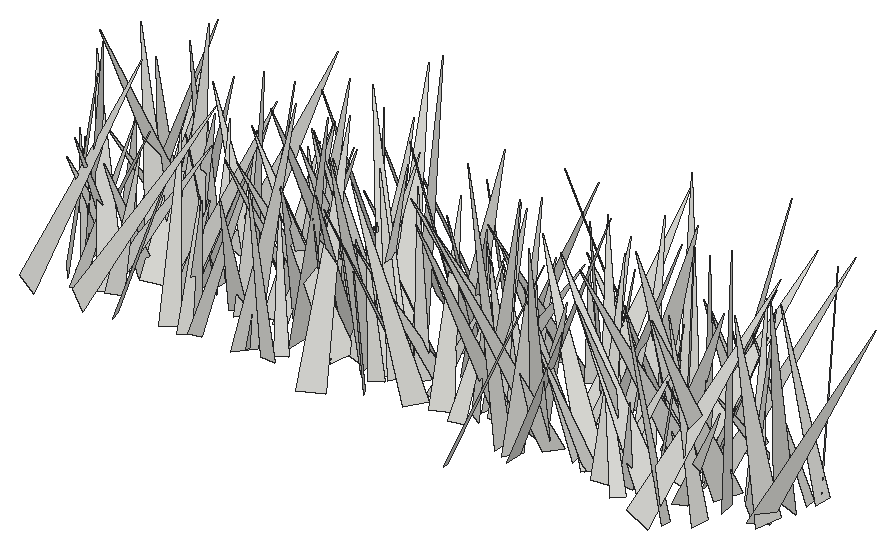
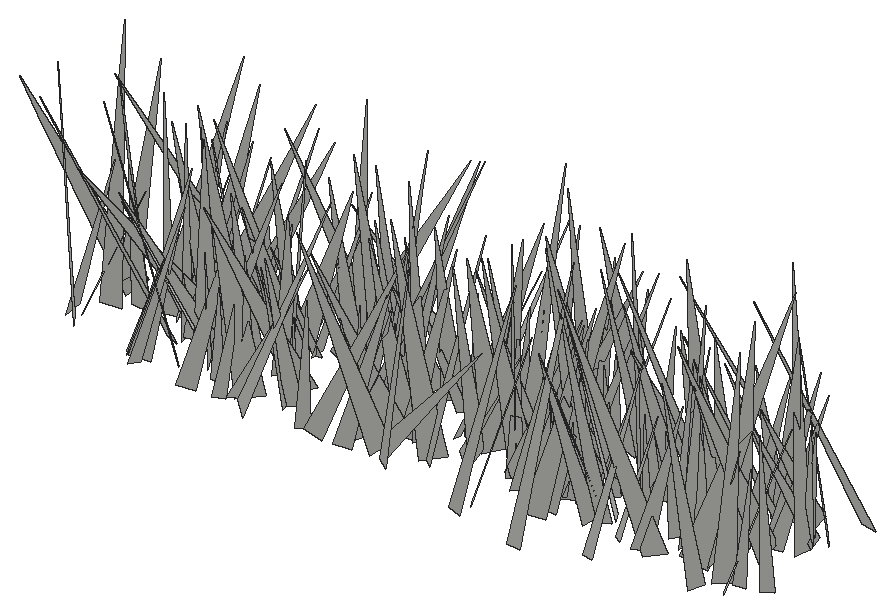
# SketchUp Ruby script. Lengths in inches.
U = 1.inch
M = Sketchup.active_model
def pt(a) = Geom::Point3d.new(a.map { |v| v * U })
def face(e, loops, mat)
  f = e.add_face(loops[0].map { |a| pt(a) })
  loops[1..].each { |l| e.add_face(l.map { |a| pt(a) }).erase! }
  f.material = f.back_material = mat if mat
  f
end
# faces: each face lists its corners as indices into pts; further lists are holes
def faces(e, pts, list, mat = nil) = list.each { |f| face(e, (f[0].is_a?(Array) ? f : [f]).map { |l| l.map { |i| pts[i] } }, mat) }
# xy, xz, yz: faces in a plane at the given z, y or x. An outline is a flat list of corners, or four numbers for a rectangle; further outlines are holes
def ring(l) = l.size == 4 ? [[l[0], l[1]], [l[2], l[1]], [l[2], l[3]], [l[0], l[3]]] : l.each_slice(2).to_a
def flat(e, list, mat, &to3) = list.each { |f| face(e, (f[0].is_a?(Array) ? f : [f]).map { |l| ring(l).map { |u, v| to3.(u, v) } }, mat) }
def xy(e, z, list, mat = nil) = flat(e, list, mat) { |x, y| [x, y, z] }
def xz(e, y, list, mat = nil) = flat(e, list, mat) { |x, z| [x, y, z] }
def yz(e, x, list, mat = nil) = flat(e, list, mat) { |y, z| [x, y, z] }
def lines(e, pts, list) = list.each { |a, b| e.add_line(pt(pts[a]), pt(pts[b])) }
# prism: a flat outline (further loops are holes) pulled along v
def prism(e, loops, v, mat = nil)
  f = face(e, loops, mat); d = Geom::Vector3d.new(v.map { |x| x * U })
  f.pushpull(f.normal.samedirection?(d) ? d.length : -d.length)
end
def box(e, o, s, mat = nil) = prism(e, [[o, [o[0] + s[0], o[1], o[2]], [o[0] + s[0], o[1] + s[1], o[2]], [o[0], o[1] + s[1], o[2]]]], [0, 0, s[2]], mat)
def at(x, y, z, deg = 0) = Geom::Transformation.translation(pt([x, y, z])) * Geom::Transformation.rotation(ORIGIN, Z_AXIS, deg.degrees)
def axes(o, x, y, z) = Geom::Transformation.new([*x, 0, *y, 0, *z, 0, *pt(o).to_a, 1])
def part(name) = M.definitions.add(name)
# library, detail: a bought-in or finely detailed component or shape, given as its bounding box
def library(name, o, s) = part(name).tap { |d| box(d.entities, o, s) }
def detail(e, o, s) = box(e.add_group.entities, o, s)
def put(e, d, t, mat = nil) = e.add_instance(d, t).tap { |i| i.material = mat if mat }
def group(e, t, mat = nil) = e.add_group.tap { |g| g.transformation = t; g.material = mat if mat }.entities
root = M.entities
c1 = part("fur_instance\#9")
p = [[0.8125,0,1.79],[0.67,-0.02,1.48],[0,-0.11,0],[0,0.11,0]]
faces(c1.entities,p,[[0,1,2,3]])
put(root,c1,axes([140.625,446.28,-27.1],[5.39727,3.08007,0.18691],[2.81936,-5.07536,2.22356],[-1.25418,1.84558,5.80286]))
put(root,c1,axes([116.41,447.99,-27.1],[4.19181,1.99584,0.5753],[1.88629,-4.2003,0.82769],[-0.86965,0.50967,4.56832]))
put(root,c1,axes([125.84,449.39,-27.1],[-1.40726,-4.75955,2.034],[-5.17479,1.24906,-0.65748],[-0.10975,2.13481,4.91949]))
put(root,c1,axes([113.78,448.04,-27.1],[4.07618,6.66518,0.05677],[6.29765,-3.82934,-2.59208],[2.18344,-1.39809,7.37028]))
put(root,c1,axes([149.72,450.49,-27.1],[0.99148,-3.49866,0.36174],[-3.47594,-0.91715,0.65665],[0.53788,0.52224,3.57665]))
put(root,c1,axes([143.02,451.46,-27.1],[-0.95701,-7.3765,1.52863],[-7.35851,1.24531,1.40248],[1.61303,1.30453,7.30491]))
put(root,c1,axes([119.95,450.31,-27.1],[3.72524,-2.31212,0.81738],[-2.32656,-3.80205,-0.15146],[-0.77532,0.29988,4.38182]))
put(root,c1,axes([120.54,448.8,-27.1],[-2.95191,2.4359,0.97471],[2.3622,3.10602,-0.60836],[1.1418,-0.12828,3.77853]))
put(root,c1,axes([110.49,447.77,-27.1],[3.27574,7.01328,0.4286],[6.91428,-3.13335,-1.57325],[1.25002,-1.04703,7.57902]))
put(root,c1,axes([144.125,451.28,-27.1],[-0.88156,-7.55851,1.51866],[-6.98391,0.13553,-3.37952],[-3.26533,1.75074,6.81814]))
put(root,c1,axes([133.73,452.16,-27.1],[-4.47092,-4.93614,0.16266],[-4.90041,4.46105,0.68268],[0.61475,-0.33851,6.62484]))
put(root,c1,axes([153.91,448.6875,-27.1],[-5.8174,-1.77979,0.63377],[-1.88895,5.44209,-2.05595],[-0.03436,2.15114,5.72563]))
put(root,c1,axes([114.86,449.83,-27.1],[-2.17172,3.54056,2.13295],[3.72846,2.71807,-0.7156],[1.78427,-1.37037,4.09143]))
put(root,c1,axes([154.72,453.05,-27.1],[4.80853,-5.64104,1.01196],[-5.19564,-4.8483,-2.3381],[-2.41883,-0.80002,7.03396]))
put(root,c1,axes([139.82,452.43,-27.1],[0.11863,-7.1905,0.64579],[-7.08435,-0.24031,-1.37429],[-1.39009,0.61104,7.05894]))
put(root,c1,axes([130.49,452.47,-27.1],[7.53052,-1.13144,2.64431],[-0.30654,-7.68469,-2.41514],[-2.85982,-2.15562,7.22191]))
put(root,c1,axes([119.4,448.99,-27.1],[3.60121,-2.60608,3.3834],[-3.59297,-4.24118,0.55747],[-2.30861,2.53545,4.41017]))
put(root,c1,axes([155.33,449.83,-27.1],[-5.94659,0.26274,1.16381],[0.1992,6.05181,-0.34844],[1.17635,0.30341,5.94219]))
put(root,c1,axes([132.16,449.81,-27.1],[-3.20539,-1.99252,1.2784],[-2.28309,3.17085,-0.78241],[0.62603,1.36182,3.69222]))
put(root,c1,axes([149.81,452.24,-27.1],[-5.8383,-2.13052,1.19785],[-1.77007,5.82456,1.73238],[1.68547,-1.263,5.96857]))
put(root,c1,axes([135.17,450.52,-27.1],[-3.75455,5.21199,1.89568],[5.51913,3.28609,1.89629],[-0.5456,-2.62523,6.13723]))
put(root,c1,axes([150.07,449.32,-27.1],[-2.40389,3.30252,0.08348],[3.28439,2.37806,0.4999],[-0.35549,-0.36124,4.05406]))
put(root,c1,axes([153.22,450.77,-27.1],[3.00481,-2.76961,0.12717],[-2.71494,-2.90128,0.96303],[0.56213,0.79222,3.97142]))
put(root,c1,axes([147.14,450.73,-27.1],[-0.30638,-3.92044,1.36874],[-3.76361,-0.31774,-1.75256],[-1.75458,1.36615,3.52026]))
put(root,c1,axes([152.52,449.32,-27.1],[3.86177,3.77021,1.4507],[3.73701,-4.09632,0.69796],[-1.5342,-0.48777,5.35169]))
put(root,c1,axes([151.61,450.49,-27.1],[-6.06762,4.08752,0.30456],[4.00596,5.79855,1.98636],[-0.86766,-1.81261,7.04117]))
put(root,c1,axes([124.23,449.36,-27.1],[6.87844,-2.02965,2.77665],[-2.6588,-7.07628,1.41394],[-2.18175,2.22463,7.03088]))
put(root,c1,axes([111.28,450.27,-27.1],[4.60486,4.04407,1.88978],[4.30358,-4.74303,-0.33665],[-1.18533,-1.50984,6.1193]))
put(root,c1,axes([113.47,452.25,-27.1],[-0.2394,-4.99537,0.47277],[-5.01072,0.21306,-0.28607],[-0.26442,0.48521,4.99291]))
put(root,c1,axes([129.92,448,-27.1],[-5.97227,4.9002,0.90124],[4.6479,5.98621,-1.7477],[1.79477,0.80344,7.52499]))
put(root,c1,axes([145.65,451.47,-27.1],[-5.30182,-0.75056,0.88287],[-0.65483,5.35184,0.61739],[0.95603,-0.49663,5.31898]))
put(root,c1,axes([111.55,452.125,-27.1],[7.9282,0.66664,2.15118],[1.11346,-8.00329,-1.62351],[-1.9576,-1.85234,7.78877]))
put(root,c1,axes([141.66,449.92,-27.1],[-7.85501,-1.13743,1.66782],[-1.3997,7.89692,-1.20666],[1.45472,1.45652,7.84468]))
put(root,c1,axes([114.93,452.67,-27.1],[3.23703,-3.40023,0.62778],[-3.13183,-3.24768,-1.44163],[-1.46538,-0.57015,4.46784]))
put(root,c1,axes([112.91,452.87,-27.1],[3.29812,-3.00828,0.87507],[-2.53709,-3.30998,-1.81667],[-1.83812,-0.82908,4.07763]))
put(root,c1,axes([121.28,452.55,-27.1],[1.53045,-4.60076,0.23907],[-4.60681,-1.52625,0.11946],[0.03806,0.26453,4.84716]))
put(root,c1,axes([152.41,448.09,-27.1],[1.49345,8.09623,0.02611],[7.76227,-1.42429,-2.34489],[2.30146,-0.44999,7.89182]))
put(root,c1,axes([114.52,449.98,-27.1],[-3.46559,5.8146,1.30946],[5.95968,3.40104,0.67057],[0.08042,-1.46897,6.73574]))
put(root,c1,axes([126.2,450.12,-27.1],[-1.47936,3.73163,0.54523],[3.76451,1.42617,0.45319],[-0.22551,-0.67216,3.98851]))
put(root,c1,axes([143.04,449.125,-27.1],[7.43701,2.08557,1.03262],[1.85087,-7.39668,1.60887],[-1.41074,1.29018,7.55449]))
put(root,c1,axes([142.72,449.47,-27.1],[-6.83852,1.49302,2.47832],[0.97247,7.17644,-1.63995],[2.72497,1.18576,6.80477]))
put(root,c1,axes([158.19,452.2,-27.1],[-6.01027,1.97565,2.91231],[2.62602,6.35479,1.10849],[2.3428,-2.05464,6.22879]))
put(root,c1,axes([128.33,451.64,-27.1],[-3.06281,-3.15709,1.43812],[-3.29391,3.24851,0.11628],[1.08883,0.94666,4.3971]))
put(root,c1,axes([127.84,454.125,-27.1],[-0.91329,-6.82842,0.06821],[-6.63421,0.90353,1.6239],[1.61843,-0.14959,6.69511]))
put(root,c1,axes([112.84,449.09,-27.1],[4.59265,0.40937,1.72839],[-0.43371,-4.3881,2.19176],[-1.72245,2.19644,4.05662]))
put(root,c1,axes([125.98,452.01,-27.1],[7.89082,-0.9052,1.78608],[-0.78265,-8.07818,-0.63641],[-1.84308,-0.44515,7.91703]))
put(root,c1,axes([141.97,452.42,-27.1],[3.60736,-4.41491,0.21347],[-4.38405,-3.53869,0.89879],[0.56311,0.73233,5.62998]))
put(root,c1,axes([151.7,453.91,-27.1],[1.64942,-7.33453,1.1804],[-6.83961,-1.97125,-2.69132],[-2.89974,0.47759,7.01946]))
put(root,c1,axes([113.76,451.03,-27.1],[3.2036,5.15972,0.63397],[4.7617,-2.61371,-2.78969],[2.08586,-1.95793,5.39475]))
put(root,c1,axes([131.92,451.17,-27.1],[-1.38179,3.78074,1.32931],[4.00762,1.30133,0.46468],[-0.00636,-1.40818,3.99842]))
put(root,c1,axes([112.24,450.73,-27.1],[0.5553,3.90242,1.15183],[3.90207,-0.84018,0.96535],[-1.15302,-0.96393,3.8217]))
put(root,c1,axes([117.9,451.76,-27.1],[1.20072,-3.47995,0.99765],[-3.52529,-0.88496,1.15597],[0.82322,1.28603,3.49507]))
put(root,c1,axes([111.97,451.16,-27.1],[0.50374,3.60666,1.32904],[3.78488,-0.69911,0.46265],[-0.67011,-1.23747,3.61216]))
put(root,c1,axes([128.89,452.07,-27.1],[-6.43604,2.78332,0.65453],[2.85741,6.20344,1.71766],[-0.1023,-1.83529,6.79846]))
put(root,c1,axes([148.56,450.65,-27.1],[0.79551,4.29487,0.6755],[4.10301,-0.51451,-1.56067],[1.4379,-0.90797,4.07959]))
put(root,c1,axes([124.49,454.31,-27.1],[6.011,-2.52803,0.45147],[-2.2406,-5.7244,-2.22212],[-1.25478,-1.8887,6.13068]))
put(root,c1,axes([153.92,453.24,-27.1],[-3.41692,-2.65793,0.41527],[-2.50813,3.39027,1.06197],[0.9728,-0.5949,4.19669]))
put(root,c1,axes([134.04,453.875,-27.1],[-4.91943,-1.92287,0.32626],[-1.70701,4.67316,1.80343],[0.9434,-1.57124,4.96446]))
put(root,c1,axes([135.52,451.55,-27.1],[0.91676,-3.52562,1.5814],[-3.59518,-0.18259,1.67709],[1.41617,1.81877,3.23385]))
put(root,c1,axes([148.35,450,-27.1],[-0.0106,6.43156,0.96228],[6.47441,-0.07994,0.60561],[-0.61077,-0.95901,6.403]))
put(root,c1,axes([138.625,451.35,-27.1],[-2.24155,-3.80564,2.54295],[-4.42537,2.52493,-0.12217],[1.16862,2.26183,4.41503]))
put(root,c1,axes([126.09,454.23,-27.1],[4.34994,-4.04005,0.73934],[-3.73736,-4.34022,-1.72779],[-1.70317,-0.79441,5.67968]))
put(root,c1,axes([147.14,450.92,-27.1],[-3.95209,5.35159,0.47213],[5.26841,3.74586,1.6413],[-1.05182,-1.34553,6.44707]))
put(root,c1,axes([121.12,449,-27.1],[5.49101,0.89671,2.25711],[-0.37206,-5.20349,2.97239],[-2.40004,2.85822,4.70322]))
put(root,c1,axes([136.73,450.76,-27.1],[-2.92394,5.35838,1.35906],[5.44647,3.05552,-0.32925],[0.94614,-1.02969,6.09534]))
put(root,c1,axes([139.3,455.6,-27.1],[-7.53778,-2.79862,0.78068],[-2.32716,7.11502,3.03655],[1.73954,-2.60846,7.44512]))
put(root,c1,axes([124.3,449.85,-27.1],[-6.72177,-1.11045,3.37602],[-2.29516,6.87097,-2.30972],[2.71346,3.06096,6.4094]))
put(root,c1,axes([157.71,454.21,-27.1],[-1.05079,-7.8114,1.55453],[-7.7743,1.34665,1.51176],[1.73053,1.30661,7.73542]))
put(root,c1,axes([125.15,455.25,-27.1],[-6.3203,-1.31951,1.76492],[-0.3807,5.93404,3.07318],[2.17051,-2.80147,5.67828]))
put(root,c1,axes([111.65,450.95,-27.1],[4.45385,0.90104,0.34779],[0.77968,-4.32278,1.21461],[-0.57002,1.12752,4.37874]))
put(root,c1,axes([138.09,453.4,-27.1],[-2.71876,-5.31687,1.33657],[-5.469,2.73415,-0.24823],[0.3815,1.3048,5.9665]))
put(root,c1,axes([138.12,450.33,-27.1],[-3.50119,3.09472,0.56001],[2.74674,3.41714,-1.71109],[1.53177,0.94611,4.34831]))
put(root,c1,axes([145.49,451.65,-27.1],[0.85166,3.52496,0.51911],[3.494,-0.72175,-0.83136],[0.69768,-0.68839,3.5298]))
put(root,c1,axes([151.67,454.3,-27.1],[3.93699,-6.31061,2.13001],[-6.14082,-4.39732,-1.67764],[-2.57895,0.83692,7.24632]))
put(root,c1,axes([117.67,451.92,-27.1],[3.41975,6.53108,1.33927],[6.45057,-2.86091,-2.51965],[1.68487,-2.30293,6.92828]))
put(root,c1,axes([123.74,455.14,-27.1],[-5.24067,-3.21189,0.67738],[-2.84495,5.08085,2.08111],[1.63749,-1.45206,5.78359]))
put(root,c1,axes([156.63,452.47,-27.1],[-3.30417,-4.76212,3.2823],[-5.25525,4.05058,0.5865],[2.41528,2.29867,5.7664]))
put(root,c1,axes([138.71,452.8125,-27.1],[6.63487,-1.65212,1.91106],[-1.73662,-6.8834,0.0785],[-1.83462,0.54083,6.83702]))
put(root,c1,axes([121.59,453.21,-27.1],[-3.32783,-6.52848,3.29816],[-6.89122,4.01297,0.99019],[2.45153,2.41834,7.26051]))
put(root,c1,axes([139.9,452.7,-27.1],[-4.97089,0.8761,1.32855],[0.91857,5.13772,0.0489],[1.29955,-0.28038,5.04727]))
put(root,c1,axes([118.82,453.8,-27.1],[-3.91635,-3.27614,1.36892],[-3.24396,4.13005,0.60351],[1.44353,0.39293,5.07017]))
put(root,c1,axes([148,451.47,-27.1],[4.12915,-1.39251,2.24683],[-2.1688,-4.1671,1.40312],[-1.51116,2.17563,4.12556]))
put(root,c1,axes([151.65,453.74,-27.1],[-5.54142,2.04017,2.02802],[2.50487,5.58649,1.22443],[1.41448,-1.90035,5.77671]))
put(root,c1,axes([139.88,451.93,-27.1],[-3.26703,2.9675,0.38966],[2.97957,3.27925,0.00816],[0.28293,-0.26806,4.41355]))
put(root,c1,axes([121.82,452.4,-27.1],[4.3952,-2.19196,2.60814],[-2.70598,-4.83259,0.49862],[-2.06997,1.6632,4.88608]))
put(root,c1,axes([123.3,453.76,-27.1],[3.09975,-1.98369,0.33098],[-1.98147,-3.11644,-0.1208],[-0.34401,0.07615,3.67817]))
put(root,c1,axes([135.15,455.39,-27.1],[6.92696,-1.79403,0.01467],[-1.72828,-6.68834,-1.86567],[-0.48147,-1.80253,6.90801]))
put(root,c1,axes([155.5,451.96,-27.1],[-6.71268,-1.89599,2.76742],[-2.51748,6.93875,-1.3526],[2.21714,2.13833,6.8429]))
put(root,c1,axes([139.75,451.75,-27.1],[0.8824,6.11345,1.2337],[6.18895,-1.01221,0.58924],[-0.77016,-1.12963,6.14863]))
put(root,c1,axes([117.23,453.05,-27.1],[-5.12716,5.45276,3.67809],[5.84452,5.9162,-0.62364],[3.01704,-2.19425,7.45865]))
put(root,c1,axes([146.11,452.62,-27.1],[7.40622,-0.19557,0.80001],[-0.28757,-7.3972,0.85392],[-0.77173,0.87956,7.35943]))
put(root,c1,axes([132.65,452.12,-27.1],[-5.52094,1.92393,0.48296],[1.85996,5.5174,-0.71721],[0.68943,0.52184,5.80241]))
put(root,c1,axes([157.79,451.82,-27.1],[6.83257,-2.01041,0.78824],[-2.1593,-6.33413,2.56189],[0.022,2.68032,6.64549]))
put(root,c1,axes([135.98,455.64,-27.1],[1.38462,-5.25865,0.1546],[-5.22749,-1.39323,-0.57157],[-0.5921,0.00308,5.40776]))
put(root,c1,axes([129.99,453.23,-27.1],[5.84499,-0.86217,1.83487],[-1.09003,-6.05756,0.62599],[-1.70936,0.91471,5.87498]))
put(root,c1,axes([149.4,455.01,-27.1],[3.81645,-5.44593,0.15233],[-5.28758,-3.65777,1.70554],[1.31259,1.09964,6.42764]))
put(root,c1,axes([116.05,454.63,-27.1],[3.45559,-4.90486,0.92565],[-4.98413,-3.32981,0.96246],[0.2699,1.30779,5.9222]))
put(root,c1,axes([118.2,453.68,-27.1],[6.4862,-0.82849,0.61771],[-0.87391,-6.49276,0.46816],[-0.55158,0.54452,6.52212]))
put(root,c1,axes([124.09,452.57,-27.1],[-0.30009,3.62925,0.24074],[3.53668,0.34756,-0.831],[0.84929,-0.16496,3.54556]))
put(root,c1,axes([115.39,456.72,-27.1],[0.76231,-8.24421,0.75454],[-8.09051,-0.90251,-1.68715],[-1.75496,0.57958,8.10565]))
put(root,c1,axes([145.42,454.12,-27.1],[-5.46396,-3.21591,2.3792],[-3.43589,5.83542,-0.00311],[2.04873,1.20967,6.3401]))
put(root,c1,axes([133.84,452.76,-27.1],[-5.20641,1.3754,0.94823],[1.21962,5.25029,-0.91901],[1.14166,0.66356,5.30602]))
put(root,c1,axes([132.34,452.26,-27.1],[-4.81407,6.51041,0.79127],[6.55623,4.75265,0.78417],[-0.16528,-1.10168,8.05889]))
put(root,c1,axes([114.375,453.07,-27.1],[1.48764,5.46016,1.29529],[5.56167,-1.25605,-1.09283],[0.74757,-1.52092,5.55267]))
put(root,c1,axes([129.38,452.38,-27.1],[1.31333,6.20143,0.89],[6.24264,-1.21867,-0.72041],[0.52849,-1.01577,6.2979]))
put(root,c1,axes([114.73,454.02,-27.1],[-4.39266,5.33205,2.64396],[5.82364,4.52851,0.54275],[1.2274,-2.40386,6.88706]))
put(root,c1,axes([149.63,455.4,-27.1],[-1.836,-5.36618,0.72675],[-5.38286,1.72484,-0.86298],[-0.59066,0.96126,5.60554]))
put(root,c1,axes([125.45,457.16,-27.1],[-0.22294,-7.81188,0.28991],[-7.80547,0.20653,-0.4373],[-0.42917,0.30182,7.80282]))
put(root,c1,axes([152.47,454.16,-27.1],[5.88559,1.89129,2.87248],[1.95642,-6.52369,0.2867],[-2.82853,-0.57687,6.17535]))
put(root,c1,axes([123.33,453.04,-27.1],[-3.03856,4.16793,1.35783],[3.96538,3.31773,-1.3102],[1.86846,-0.26309,4.98878]))
put(root,c1,axes([128.83,455.48,-27.1],[2.48728,-3.44318,0.65298],[-3.47724,-2.52444,-0.0662],[-0.43662,0.49004,4.24707]))
put(root,c1,axes([127.87,454.65,-27.1],[-1.21907,-3.82959,1.50139],[-4.09681,0.98993,-0.80143],[-0.36895,1.66143,3.93822]))
put(root,c1,axes([115.7,452.12,-27.1],[-3.21539,5.33291,0.27404],[5.21793,3.20577,-1.16191],[1.13501,0.36996,6.11789]))
put(root,c1,axes([140.24,453.99,-27.1],[-3.96056,0.86775,0.15545],[0.85071,3.94968,-0.37345],[0.23119,0.33194,4.03727]))
put(root,c1,axes([141.125,453.48,-27.1],[-3.9297,0.38452,0.60241],[0.18265,3.7953,-1.23109],[0.69093,1.18368,3.75164]))
put(root,c1,axes([117.01,455.4,-27.1],[-6.68895,-1.28776,2.75903],[-1.15,7.23488,0.5888],[2.81923,-0.10417,6.78629]))
put(root,c1,axes([137.38,454.17,-27.1],[4.47757,-3.00826,2.16701],[-3.51648,-4.52249,0.98776],[-1.1747,2.07164,5.30307]))
put(root,c1,axes([118.74,454.07,-27.1],[-5.92753,-0.80933,1.51712],[-1.07571,5.99367,-1.00549],[1.34146,1.2301,5.89742]))
put(root,c1,axes([129.59,454.55,-27.1],[4.46233,4.90899,2.88894],[5.22756,-4.98695,0.39938],[-2.26203,-1.84084,6.62202]))
put(root,c1,axes([132.49,455.4,-27.1],[-2.45002,-3.17903,0.27674],[-3.09062,2.27713,-1.20338],[-0.79426,0.94543,3.82893]))
put(root,c1,axes([153.06,453.02,-27.1],[4.06306,2.1594,0.43468],[1.91332,-3.91175,1.54848],[-1.0914,1.18135,4.33286]))
put(root,c1,axes([156.21,453.49,-27.1],[-0.40963,5.6712,0.85204],[5.69515,0.30195,0.72827],[-0.67361,-0.89587,5.63914]))
put(root,c1,axes([114.55,455.33,-27.1],[3.71133,-3.4553,1.19556],[-3.62183,-3.7076,0.52772],[-0.50083,1.20708,5.04327]))
put(root,c1,axes([153.89,457.5625,-27.1],[-3.33896,-2.6162,0.26799],[-2.1089,2.92233,2.25332],[1.57125,-1.6372,3.59384]))
put(root,c1,axes([124.94,455.46,-27.1],[2.55776,-3.86723,2.22173],[-4.13899,-3.01226,-0.47827],[-1.66143,1.55064,4.61182]))
put(root,c1,axes([129.2,454.25,-27.1],[-3.21117,5.73542,2.2751],[5.803,3.67883,-1.08356],[2.09673,-1.39782,6.48325]))
put(root,c1,axes([128.78,455.6,-27.1],[-0.87207,-5.64239,2.10409],[-5.67136,0.05471,-2.20385],[-2.02471,2.277,5.26688]))
put(root,c1,axes([127.8,456.39,-27.1],[-5.01187,1.13995,1.85475],[1.60842,5.07616,1.22637],[1.46717,-1.67079,4.99142]))
put(root,c1,axes([121.78,455.43,-27.1],[5.2265,3.38981,1.10604],[3.55749,-5.09026,-1.20993],[-0.2416,-1.62138,6.11091]))
put(root,c1,axes([123.86,455.46,-27.1],[1.63751,6.97927,2.94123],[7.53115,-1.18196,-1.38823],[0.80173,-3.15202,7.03309]))
put(root,c1,axes([136.96,455.32,-27.1],[4.24231,-3.44067,0.07958],[-3.18347,-3.87509,2.16585],[1.3077,1.72835,5.01442]))
put(root,c1,axes([145.77,454.19,-27.1],[-5.07407,3.61415,0.85454],[3.5922,5.14344,-0.42375],[0.94256,-0.14624,6.2152]))
put(root,c1,axes([126.96,454.25,-27.1],[1.83922,3.08635,0.93557],[2.6886,-2.06216,1.51739],[-1.78108,0.07419,3.25666]))
put(root,c1,axes([133.74,456.9,-27.1],[-4.39451,-5.32367,1.29551],[-5.40377,4.48556,0.10243],[0.905,0.93264,6.90237]))
put(root,c1,axes([158.61,455.26,-27.1],[-4.94313,-1.68267,0.02369],[-1.64372,4.81198,-1.18726],[-0.36076,1.13137,5.08492]))
put(root,c1,axes([112.91,453.41,-27.1],[7.28027,0.47928,1.68125],[-0.05604,-7.13268,2.27604],[-1.74733,2.22571,6.93193]))
put(root,c1,axes([126.48,455.95,-27.1],[0.21554,-5.31829,2.18174],[-5.56977,-0.73327,-1.23719],[-1.42193,2.0661,5.17688]))
put(root,c1,axes([149.51,455.93,-27.1],[5.6621,3.46946,2.68851],[3.90579,-5.98471,-0.5026],[-2.00251,-1.86297,6.62147]))
put(root,c1,axes([112.05,458.35,-27.1],[-3.67716,-3.23058,0.06887],[-2.92053,3.36739,2.02339],[1.38271,-1.47883,4.45691]))
put(root,c1,axes([125.39,458.07,-27.1],[2.94915,-5.28887,0.70098],[-5.06545,-3.02722,-1.5291],[-1.67475,-0.15728,5.85931]))
put(root,c1,axes([110.33,456.74,-27.1],[0.87128,-4.23502,0.75689],[-4.24446,-0.72019,0.85631],[0.702,0.90186,4.23807]))
put(root,c1,axes([148.21,453.83,-27.1],[-1.0825,6.58238,0.66021],[6.6005,1.02978,0.55528],[-0.44383,-0.73975,6.64764]))
put(root,c1,axes([120.27,457.22,-27.1],[-1.91573,-3.10975,0.18965],[-3.07242,1.92263,0.49017],[0.51647,-0.09744,3.61944]))
put(root,c1,axes([112.78,457.46,-27.1],[5.63565,-3.00774,1.4531],[-2.80235,-5.80815,-1.15361],[-1.81792,-0.37081,6.28301]))
put(root,c1,axes([114.55,456.28,-27.1],[-3.7389,-0.44853,0.79303],[-0.43438,3.82202,0.11371],[0.80087,-0.02096,3.764]))
put(root,c1,axes([145.53,457.43,-27.1],[3.43501,-7.39782,1.03394],[-7.28345,-3.06455,2.27067],[1.65774,1.86463,7.83397]))
put(root,c1,axes([148.88,458.74,-27.1],[3.46816,-3.92613,0.03464],[-3.68547,-3.27126,-1.77763],[-1.35388,-1.15247,4.92774]))
put(root,c1,axes([159.02,455.84,-27.1],[-5.68888,-0.08485,0.69236],[-0.12916,5.71868,-0.36046],[0.68548,0.37338,5.67808]))
put(root,c1,axes([152.85,457.79,-27.1],[1.51534,-5.37644,0.92666],[-5.31705,-1.67082,-0.99923],[-1.22223,0.60275,5.49581]))
put(root,c1,axes([122.02,456.33,-27.1],[0.68635,-5.64905,2.27441],[-5.90756,-0.06201,1.6287],[1.47832,2.3749,5.45254]))
put(root,c1,axes([150.66,454.125,-27.1],[5.57667,1.59527,0.3002],[1.43066,-5.3377,1.78788],[-0.76695,1.64269,5.51794]))
put(root,c1,axes([140.3,458.54,-27.1],[-0.06223,-5.95217,0.13196],[-5.73579,0.02457,-1.59678],[-1.59576,0.14382,5.73432]))
put(root,c1,axes([123.22,455.02,-27.1],[3.32598,3.77438,0.4675],[3.78797,-3.34308,0.04133],[-0.34022,-0.32329,5.03054]))
put(root,c1,axes([158.22,456.73,-27.1],[-5.21121,-4.35385,3.58957],[-4.50193,6.15376,0.92827],[3.40202,1.4741,6.72689]))
put(root,c1,axes([151.75,453.91,-27.1],[4.07971,3.91858,0.07723],[3.79656,-3.97882,1.32677],[-0.97331,0.90496,5.499]))
put(root,c1,axes([150.89,454.4,-27.1],[-0.59735,8.07244,1.41711],[8.08686,0.34954,1.4177],[-1.33238,-1.49761,7.96939]))
put(root,c1,axes([117.91,455.06,-27.1],[-3.18277,2.93848,0.48438],[2.88307,3.21784,-0.5768],[0.74643,0.10079,4.29324]))
put(root,c1,axes([131.42,453.61,-27.1],[-6.0602,5.67803,0.65626],[5.53411,6.06799,-1.39639],[1.4298,0.57987,8.18634]))
put(root,c1,axes([133.57,456.53,-27.1],[4.4224,-5.22883,1.99199],[-5.58659,-4.26873,1.19762],[-0.31423,2.30295,6.7427]))
put(root,c1,axes([151.49,452.56,-27.1],[-3.48939,6.7058,0.49493],[5.71017,3.24965,-3.77124],[3.55058,1.36403,6.55144]))
put(root,c1,axes([146.32,456.58,-27.1],[-3.33469,1.40616,1.82105],[1.56398,3.73727,-0.02186],[1.68745,-0.685,3.61897]))
put(root,c1,axes([138.22,458.57,-27.1],[2.83348,-4.00549,0.52306],[-3.76222,-2.8494,-1.43972],[-1.47079,-0.42795,4.69039]))
put(root,c1,axes([152.75,455.13,-27.1],[4.68977,6.59581,0.10077],[6.41242,-4.52929,-1.96857],[1.54784,-1.22048,7.85006]))
put(root,c1,axes([122.61,456.62,-27.1],[4.92372,-1.23429,0.65682],[-1.32256,-4.89156,0.72207],[-0.45359,0.86432,5.02445]))
put(root,c1,axes([146.79,458.5,-27.1],[3.04717,-2.22298,0.43436],[-2.028,-3.00193,-1.13631],[-1.00873,-0.67996,3.59662]))
put(root,c1,axes([111.84,457.25,-27.1],[0.6335,-3.36408,1.34348],[-3.58683,-0.77327,-0.24494],[-0.50657,1.2682,3.41444]))
put(root,c1,axes([128.84,459.18,-27.1],[-3.83157,-3.11067,0.41222],[-2.87249,3.73899,1.51524],[1.26294,-0.9332,4.69694]))
put(root,c1,axes([152.77,458.34,-27.1],[-4.67386,-0.0885,1.27111],[0.2568,4.66814,1.26925],[1.24804,-1.29194,4.49909]))
put(root,c1,axes([143.4375,456.88,-27.1],[4.00682,1.30969,1.18737],[1.29487,-4.17692,0.23764],[-1.20352,-0.13365,4.20874]))
put(root,c1,axes([120.3,459.8,-27.1],[-2.61623,-5.06997,0.16776],[-4.93297,2.58676,1.24576],[1.18261,-0.42604,5.56752]))
put(root,c1,axes([146.1,457.97,-27.1],[-4.58905,2.11277,0.48874],[2.15665,4.32669,1.54618],[-0.22698,-1.60562,4.80963]))
put(root,c1,axes([138,457.09,-27.1],[3.18405,-1.52738,1.26596],[-1.78098,-3.25535,0.55182],[-0.87386,1.06936,3.48806]))
put(root,c1,axes([118.55,457.38,-27.1],[-3.73959,3.61146,1.09906],[3.77498,3.58144,1.07604],[0.00944,-1.53809,5.08619]))
put(root,c1,axes([131.83,454.9,-27.1],[-7.99125,0.08509,2.25297],[-0.74491,7.73167,-2.93422],[2.12796,3.02611,7.43355]))
put(root,c1,axes([143.01,456.74,-27.1],[-1.4542,4.67664,1.33998],[4.76533,1.65076,-0.58976],[0.97884,-1.08869,4.86188]))
put(root,c1,axes([135.36,458.67,-27.1],[-3.25628,-4.53556,1.56998],[-4.60157,3.48952,0.53691],[1.36443,0.94415,5.55755]))
put(root,c1,axes([117.53,457.38,-27.1],[1.82991,-7.19945,3.13467],[-7.38413,-0.48301,3.20126],[2.67073,3.59742,6.70317]))
put(root,c1,axes([153.86,457.45,-27.1],[-3.57996,-1.2077,0.30439],[-1.24532,3.48547,-0.8173],[0.0195,0.87192,3.68872]))
put(root,c1,axes([151.1875,456.66,-27.1],[5.81873,5.70667,1.51485],[5.84557,-5.86726,-0.35074],[-0.83073,-1.31442,8.14252]))
put(root,c1,axes([145.125,458.73,-27.1],[-5.01465,-5.39389,0.78065],[-5.43536,4.87162,-1.25473],[-0.40033,1.42249,7.25716]))
put(root,c1,axes([143.71,454.99,-27.1],[-2.62249,6.7547,0.84995],[6.3246,2.75431,-2.37468],[2.5195,0.11678,6.84575]))
put(root,c1,axes([147.95,457.22,-27.1],[-0.46969,3.55211,0.73396],[3.59032,0.35011,0.60316],[-0.51554,-0.79795,3.53189]))
put(root,c1,axes([129.05,460.33,-27.1],[-2.89154,-5.8907,0.51675],[-5.81601,2.937,0.93617],[1.06836,0.04534,6.49499]))
put(root,c1,axes([141.16,458.32,-27.1],[1.90593,-3.10212,1.28599],[-3.27722,-2.04084,-0.06594],[-0.73267,1.05893,3.64024]))
put(root,c1,axes([136.35,457.3,-27.1],[-4.35257,-4.39527,0.35538],[-3.69396,3.36161,-3.66659],[-2.40819,2.78761,4.98191]))
put(root,c1,axes([124.13,461.42,-27.1],[-3.49524,-7.20934,0.56433],[-6.86604,3.50524,2.25399],[2.26947,-0.49846,7.68835]))
put(root,c1,axes([113.61,458.75,-27.1],[5.71322,-0.96407,0.62556],[-0.92485,-5.73993,-0.39936],[-0.68221,-0.29224,5.7802]))
put(root,c1,axes([136.45,457.51,-27.1],[6.61677,-1.08212,0.53072],[-1.15649,-6.53431,1.0953],[-0.3394,1.16883,6.6146]))
